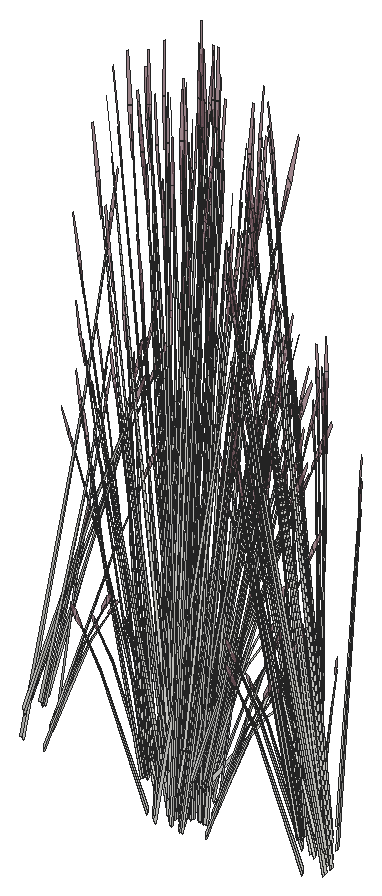
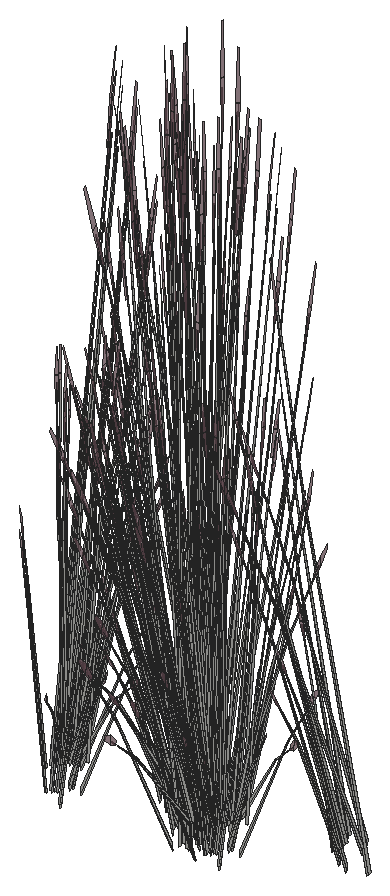
# SketchUp Ruby script. Lengths in inches.
U = 1.inch
M = Sketchup.active_model
def pt(a) = Geom::Point3d.new(a.map { |v| v * U })
def face(e, loops, mat)
  f = e.add_face(loops[0].map { |a| pt(a) })
  loops[1..].each { |l| e.add_face(l.map { |a| pt(a) }).erase! }
  f.material = f.back_material = mat if mat
  f
end
# faces: each face lists its corners as indices into pts; further lists are holes
def faces(e, pts, list, mat = nil) = list.each { |f| face(e, (f[0].is_a?(Array) ? f : [f]).map { |l| l.map { |i| pts[i] } }, mat) }
# xy, xz, yz: faces in a plane at the given z, y or x. An outline is a flat list of corners, or four numbers for a rectangle; further outlines are holes
def ring(l) = l.size == 4 ? [[l[0], l[1]], [l[2], l[1]], [l[2], l[3]], [l[0], l[3]]] : l.each_slice(2).to_a
def flat(e, list, mat, &to3) = list.each { |f| face(e, (f[0].is_a?(Array) ? f : [f]).map { |l| ring(l).map { |u, v| to3.(u, v) } }, mat) }
def xy(e, z, list, mat = nil) = flat(e, list, mat) { |x, y| [x, y, z] }
def xz(e, y, list, mat = nil) = flat(e, list, mat) { |x, z| [x, y, z] }
def yz(e, x, list, mat = nil) = flat(e, list, mat) { |y, z| [x, y, z] }
def lines(e, pts, list) = list.each { |a, b| e.add_line(pt(pts[a]), pt(pts[b])) }
# prism: a flat outline (further loops are holes) pulled along v
def prism(e, loops, v, mat = nil)
  f = face(e, loops, mat); d = Geom::Vector3d.new(v.map { |x| x * U })
  f.pushpull(f.normal.samedirection?(d) ? d.length : -d.length)
end
def box(e, o, s, mat = nil) = prism(e, [[o, [o[0] + s[0], o[1], o[2]], [o[0] + s[0], o[1] + s[1], o[2]], [o[0], o[1] + s[1], o[2]]]], [0, 0, s[2]], mat)
def at(x, y, z, deg = 0) = Geom::Transformation.translation(pt([x, y, z])) * Geom::Transformation.rotation(ORIGIN, Z_AXIS, deg.degrees)
def axes(o, x, y, z) = Geom::Transformation.new([*x, 0, *y, 0, *z, 0, *pt(o).to_a, 1])
def part(name) = M.definitions.add(name)
# library, detail: a bought-in or finely detailed component or shape, given as its bounding box
def library(name, o, s) = part(name).tap { |d| box(d.entities, o, s) }
def detail(e, o, s) = box(e.add_group.entities, o, s)
def put(e, d, t, mat = nil) = e.add_instance(d, t).tap { |i| i.material = mat if mat }
def group(e, t, mat = nil) = e.add_group.tap { |g| g.transformation = t; g.material = mat if mat }.entities
root = M.entities
M.materials.add("LightPink_Translucent").color = [144, 107, 117]
M.materials["LightPink_Translucent"].alpha = 0.75
c1 = part("blade")
p = [[2.15,0.21,22],[0,0.17,0],[0.09,0.45,0],[2.18,0.31,22],[2.29,0.31,22],[0.38,0.45,0],
  [2.48,0.24,33],[2.49,0.24,33],[2.48,0.22,33]]
faces(c1.entities,p,[[0,1,2,3],[4,5,2,3],[6,3,4,7],[8,0,3,6]])
c2 = part("seeds")
p = [[0.3,-0.1,1.38],[-0.01,-0.03,1.59],[-0.01,-0.03,0.03],[0.14,-0.07,-0.07],[0.29,-0.03,3],[0.15,0.01,3.11]]
faces(c2.entities,p,[[0,1,2,3],[1,0,4,5]],"LightPink_Translucent")
c3 = part("blade with seeds")
put(c3.entities,c1,at(0,0,0))
put(c3.entities,c2,axes([2.4,0.25,30.99],[1.5799,-0.05474,1.17369],[-0.12525,1.92788,0.29478],[-0.07173,-0.02425,1.56792]))
put(root,c3,axes([249.3,462.4375,653.93],[-0.09617,-0.45271,-0.03492],[0.45453,-0.10408,-0.15832],[0.09492,0.0287,0.52218]))
put(root,c3,axes([247.53,460.36,652.06],[0.52267,0.08829,-0.62353],[-0.11029,0.54463,-0.16365],[0.15598,0.06599,1.37633]))
put(root,c3,axes([247.42,461.52,653.875],[-0.18664,-0.09279,1.71376],[0.38624,-0.38925,0.13857],[0.24072,0.1756,0.73262]))
put(root,c3,axes([248.45,462.39,654.53],[0.28589,0.33718,-0.35414],[-0.32644,0.31919,0.4572],[0.16586,0.04856,0.87481]))
put(root,c3,axes([249.84,461.31,652.77],[-0.31044,0.08891,1.1486],[0.14613,-0.36744,0.84392],[0.16469,0.02514,0.25299]))
put(root,c3,axes([248.95,461.22,654.53],[0.41757,0.15024,-0.35414],[-0.12179,0.4383,0.4572],[0.16812,-0.04019,0.87481]))
put(root,c3,axes([248.15,462.16,654.98],[0.50227,0.01297,-0.71045],[-0.03373,0.54602,0.08574],[0.21278,0.05762,1.00501]))
put(root,c3,axes([249.52,460.8,651.49],[-0.02626,-0.08176,1.76342],[0.18213,-0.47826,-0.26939],[0.18372,-0.00688,0.30037]))
put(root,c3,axes([247.82,460.67,653.875],[-0.20841,0.0122,1.71376],[0.13825,-0.52864,0.13857],[0.297,0.0327,0.73262]))
put(root,c3,axes([248.58,461.17,654.98],[0.44151,-0.23785,-0.71045],[0.24605,0.4896,0.08574],[0.21333,-0.05562,1.00501]))
put(root,c3,axes([249.26,461.9,652.59],[-0.12101,-0.13245,1.43002],[0.15744,-0.43816,-0.30754],[0.24483,0.05936,0.61141]))
put(root,c3,axes([259.18,461,651.875],[0.17434,-0.11391,1.71376],[0.14677,0.52637,0.13857],[-0.27369,0.11897,0.73262]))
put(root,c3,axes([258.63,461.89,650.59],[0.17462,0.04421,1.43002],[0.11254,0.45156,-0.30754],[-0.23719,0.08453,0.61141]))
put(root,c3,axes([260.18,460.45,651.34],[0.14282,-0.0779,1.77064],[0.04925,0.54394,0.13857],[-0.30935,0.07218,0.63284]))
put(root,c3,axes([258.64,460.8125,652.72],[-0.08205,0.06992,1.74944],[0.00698,0.51086,-0.27667],[-0.18807,0.06644,0.14031]))
put(root,c3,axes([258.9,460.52,652.53],[-0.41757,-0.15024,-0.35414],[0.12179,-0.4383,0.4572],[-0.16812,0.04019,0.87481]))
put(root,c3,axes([257.73,461.33,652.71],[0.06412,0.01444,1.77383],[0.19837,0.47583,-0.16761],[-0.13126,0.12489,0.31391]))
put(root,c3,axes([259.19,460.74,652.68],[-0.13612,0.48987,-0.51099],[-0.46669,-0.16791,-0.3958],[-0.1879,0.04492,0.97773]))
put(root,c3,axes([258.96,460.71,649.49],[0.01274,0.08487,1.76342],[-0.25688,0.44323,-0.26939],[-0.18246,-0.02234,0.30037]))
put(root,c3,axes([258.27,462.84,650.77],[0.2094,-0.24408,1.1486],[0.08263,0.38639,0.84392],[-0.15132,0.06919,0.25299]))
put(root,c3,axes([259,460.46,652.73],[0.14195,-0.49104,0.48003],[0.46669,0.16791,0.3958],[-0.18353,0.02951,0.9933]))
put(root,c3,axes([259.17,460.32,653.03],[0.25281,0.48765,-0.1216],[-0.44869,0.23964,-0.67495],[-0.18908,0.06434,1.02557]))
put(root,c3,axes([258.97,460.33,652.73],[-0.18454,-0.3672,0.0643],[0.33652,-0.17973,0.50621],[-0.14834,0.03546,0.77189]))
put(root,c3,axes([259.8125,461.35,651.875],[0.1255,-0.16547,1.71376],[0.31687,0.44665,0.13857],[-0.21734,0.2034,0.73262]))
put(root,c3,axes([259.06,461.78,652.53],[-0.43736,0.07697,-0.35414],[-0.11549,-0.43998,0.4572],[-0.12533,0.11818,0.87481]))
put(root,c3,axes([258.82,463.09,649.49],[0.0674,0.0538,1.76342],[0.11428,0.49852,-0.26939],[-0.14937,0.10631,0.30037]))
put(root,c3,axes([259.11,461.6875,652.73],[-0.12461,-0.49565,0.48003],[0.48882,-0.08602,0.3958],[-0.14406,0.11657,0.9933]))
put(root,c3,axes([259.02,461.59,652.73],[-0.34493,-0.22649,0.0643],[0.20082,-0.32253,0.50621],[-0.11059,0.10427,0.77189]))
put(root,c3,axes([259.72,461.76,651.875],[0.09355,-0.18511,1.71376],[0.39247,0.38307,0.13857],[-0.17705,0.23875,0.73262]))
put(root,c3,axes([259.34,460.47,653.05],[0.41757,0.15024,0.35414],[-0.12179,0.4383,-0.4572],[-0.16812,0.04019,0.87481]))
put(root,c3,axes([259.42,461.83,652.68],[0.12908,0.49174,-0.51099],[-0.48882,0.08602,-0.3958],[-0.14008,0.13208,0.97773]))
put(root,c3,axes([258.65,462.72,652.72],[-0.01249,0.10657,1.74944],[0.35444,0.37075,-0.27667],[-0.09279,0.17532,0.14031]))
put(root,c3,axes([260.64,461.48,650.06],[-0.52267,-0.08829,-0.62353],[0.11029,-0.54463,-0.16365],[-0.15598,-0.06599,1.37633]))
put(root,c3,axes([259.95,462.51,650.02],[-0.47024,-0.26927,-0.49651],[0.28107,-0.48284,0],[-0.1071,-0.06133,1.57504]))
put(root,c3,axes([259.1875,461.48,653.03],[0.46478,0.29695,-0.1216],[-0.26776,0.43004,-0.67495],[-0.13131,0.14949,1.02557]))
put(root,c3,axes([260.24,462.84,650.375],[-0.31414,0.53965,0],[-0.52557,-0.30095,-0.51607],[-0.1197,-0.06854,1.63711]))
put(root,c3,axes([258.42,462.77,653.65],[0.44338,0.14375,-0.06488],[-0.13639,0.44245,-0.29416],[-0.07252,0.06718,0.97024]))
put(root,c3,axes([259.41,461.52,653.05],[0.43736,-0.07697,0.35414],[0.11549,0.43998,-0.4572],[-0.12533,0.11818,0.87481]))
put(root,c3,axes([259.66,463.62,650.59],[0.15856,-0.08496,1.43002],[0.39147,0.25616,-0.30754],[-0.11652,0.22165,0.61141]))
put(root,c3,axes([261.23,461.5625,650.67],[-0.5073,0.35754,-0.29095],[-0.33735,-0.5052,-0.50002],[-0.12516,-0.05131,1.59708]))
put(root,c3,axes([259.83,462.69,652.73],[-0.35779,-0.36745,0.48003],[0.37996,-0.3169,0.3958],[-0.066,0.17239,0.9933]))
put(root,c3,axes([260.08,462.3125,650.03],[-0.11803,-0.46926,-0.30978],[0.46876,-0.13325,0.30978],[-0.0945,-0.05411,1.38974]))
put(root,c3,axes([259.7,462.66,652.73],[-0.4129,-0.02509,0.0643],[0.01132,-0.37891,0.50621],[-0.04321,0.14514,0.77189]))
put(root,c3,axes([259.83,462.8,652.53],[-0.33997,0.28354,-0.35414],[-0.32182,-0.32376,0.4572],[-0.04897,0.1645,0.87481]))
put(root,c3,axes([261.57,461.95,650.06],[-0.33843,0.40479,-0.62353],[-0.42041,-0.36705,-0.16365],[-0.13561,0.10098,1.37633]))
put(root,c3,axes([258.62,463.8125,652.71],[0.057,-0.03251,1.77383],[0.47114,0.21627,-0.16761],[-0.01107,0.18007,0.31391]))
put(root,c3,axes([261.8,461.73,650.46],[-0.49063,-0.43346,-0.25192],[0.41285,-0.48673,0.5513],[-0.13212,0.05071,1.68216]))
put(root,c3,axes([260.05,462.5,653.34],[-0.01307,0.49815,-0.7886],[-0.55054,-0.03346,0.09517],[-0.0581,0.21104,1.11556]))
put(root,c3,axes([260.04,463.9,650.77],[-0.013,-0.32022,1.1486],[0.32493,0.22839,0.84392],[-0.0639,0.15263,0.25299]))
put(root,c3,axes([261.55,461.63,650.21],[-0.54562,0.03324,-0.44739],[-0.04934,-0.55185,0.21531],[-0.09768,0.05593,1.43643]))
put(root,c3,axes([260.51,462.56,650.48],[0.47024,0.26927,0.49651],[-0.28107,0.48284,0],[-0.1071,-0.06133,1.57504]))
put(root,c3,axes([259.87,463.2,651.36],[0.01104,-0.27801,1.54345],[0.49652,0.14685,0.21329],[-0.04302,0.2963,0.72882]))
put(root,c3,axes([261.18,461.72,650.62],[-0.09693,0.48062,0.1448],[-0.47357,-0.08343,-0.41347],[-0.08619,-0.04935,1.26744]))
put(root,c3,axes([262.125,463.06,650.02],[-0.47024,0.26927,-0.49651],[-0.28107,-0.48284,0],[-0.1071,0.06133,1.57504]))
put(root,c3,axes([262.16,462.91,650.19],[-0.31023,-0.54153,-0.05142],[0.52557,-0.30095,0.51607],[-0.12951,0.05156,1.6363]))
put(root,c3,axes([260.17,462.67,653],[0.35968,0.36185,-0.5672],[-0.37996,0.3169,-0.43934],[-0.05473,0.18385,1.08528]))
put(root,c3,axes([262.01,462.84,650.03],[-0.46876,-0.13325,-0.30978],[0.11803,-0.46926,0.30978],[-0.0945,0.05411,1.38974]))
put(root,c3,axes([260,462.4,653.05],[0.33997,-0.28354,0.35414],[0.32182,0.32376,-0.4572],[-0.04897,0.1645,0.87481]))
put(root,c3,axes([262.28,460.84,650.84],[-0.01373,-0.50706,1.41272],[0.62119,0.13144,0.59816],[-0.14692,0.27746,1.3335]))
put(root,c3,axes([259.79,462.48,653.4],[0.55221,0.02668,-0.13498],[-0.01509,0.50521,-0.74919],[-0.03836,0.19458,1.13838]))
put(root,c3,axes([259.77,463.21,650.82],[0.45645,-0.09537,0.06507],[0.10494,0.38421,-0.86304],[-0.02894,0.19449,0.7736]))
put(root,c3,axes([261.93,461.48,650.67],[0.05855,0.61451,-0.29095],[-0.60981,0.03716,-0.50002],[-0.10738,0.08185,1.59708]))
put(root,c3,axes([260.57,462.15,651.875],[-0.0123,-0.2067,1.71376],[0.53301,0.13712,0.13857],[-0.03297,0.29456,0.73262]))
put(root,c3,axes([261.03,461.26,650.36],[0.63506,0.11347,0.45755],[-0.12924,0.64083,0.17955],[-0.09281,-0.06188,1.58856]))
put(root,c3,axes([260.68,462.28,650.47],[0.53992,-0.14294,0.17642],[0.13332,0.53195,0.35086],[-0.04815,-0.07751,1.60407]))
put(root,c3,axes([261.38,462.37,650.2],[-0.50654,-0.24178,0],[0.24378,-0.50239,0],[0,0,1.62707]))
put(root,c3,axes([262.55,462.97,650.375],[0.31414,0.53965,0],[-0.52557,0.30095,-0.51607],[-0.1197,0.06854,1.63711]))
put(root,c3,axes([260.95,463.21,653.0625],[-0.4951,-0.14079,0.53283],[0.1693,-0.46287,0.43934],[0.02975,0.18203,1.10256]))
put(root,c3,axes([260.82,463.24,652.73],[-0.37023,0.18303,0.0643],[-0.18122,-0.33376,0.50621],[0.03575,0.14712,0.77189]))
put(root,c3,axes([262.29,462.3125,650.47],[0.14515,-0.53522,0.17642],[0.53115,0.15146,0.35086],[-0.09175,0.00261,1.60407]))
put(root,c3,axes([262.05,461.6,650.62],[0.37121,0.32357,0.1448],[-0.30963,0.36505,-0.41347],[-0.08619,0.04935,1.26744]))
put(root,c3,axes([261.91,461.2,650.3],[-0.46736,-0.46353,-0.06131],[0.46764,-0.46381,0],[-0.01632,-0.01619,1.75571]))
put(root,c3,axes([262.04,461.37,650.72],[0.54562,-0.03324,0.44739],[0.04934,0.55185,-0.21531],[-0.09768,0.05593,1.43643]))
put(root,c3,axes([262.17,462.63,650.33],[0.62903,0.17504,0.30756],[-0.15737,0.62568,-0.36492],[-0.10411,0.07831,1.64885]))
put(root,c3,axes([262.44,462.6,650.48],[0.47024,-0.26927,0.49651],[0.28107,0.48284,0],[-0.1071,0.06133,1.57504]))
put(root,c3,axes([261.49,462.16,650.2],[-0.16394,-0.4643,0],[0.46814,-0.1626,0],[0,0,1.54371]))
put(root,c3,axes([260.9,463.14,649.49],[0.08132,-0.0293,1.76342],[0.48914,0.1613,-0.26939],[0.0143,0.18179,0.30037]))
put(root,c3,axes([261.01,463.3,652.53],[-0.15148,0.41415,-0.35414],[-0.44193,-0.12079,0.4572],[0.04052,0.16674,0.87481]))
put(root,c3,axes([262.16,461.24,650.21],[-0.24378,0.48527,-0.44739],[-0.50654,-0.23354,0.21531],[0,0.11186,1.43643]))
put(root,c3,axes([260.69,464.04,652.72],[0.06369,0.08672,1.74944],[0.51399,0.03407,-0.27667],[0.05169,0.19126,0.14031]))
put(root,c3,axes([263.12,460.95,650.47],[-0.39477,-0.39228,0.17642],[0.39783,-0.38049,0.35086],[-0.0436,0.08011,1.60407]))
put(root,c3,axes([261.76,460.72,650.21],[0,-0.62313,0],[0.62828,0,0],[0,0,1.79456]))
put(root,c3,axes([262.07,460.97,650.29],[0,0.62282,-0.05637],[-0.62828,0,0],[0,0.01957,1.79368]))
put(root,c3,axes([260.96,462.87,653.05],[0.15148,-0.41415,0.35414],[0.44193,0.12079,-0.4572],[0.04052,0.16674,0.87481]))
put(root,c3,axes([260.74,459.52,650.47],[-0.14515,0.53522,0.17642],[-0.53115,-0.15146,0.35086],[0.09175,-0.00261,1.60407]))
put(root,c3,axes([261.77,462.18,650.29],[0.21845,0.61869,-0.06012],[-0.62418,0.21679,0],[0.00763,0.02161,1.72173]))
put(root,c3,axes([261.05,462.93,652.98],[0.23981,0.43789,-0.71045],[-0.49365,0.24404,0.08574],[0.05608,0.21158,1.00501]))
put(root,c3,axes([263.58,461.36,650.2],[-0.62797,-0.00431,-0.04976],[0,-0.6019,0.49943],[-0.01973,0.13702,1.58352]))
put(root,c3,axes([262.34,459.55,650.47],[-0.53992,0.14294,0.17642],[-0.13332,-0.53195,0.35086],[0.04815,0.07751,1.60407]))
put(root,c3,axes([261.55,464.34,653.65],[0.34721,-0.30895,-0.06488],[0.31814,0.33837,-0.29416],[0.0224,0.09588,0.97024]))
put(root,c3,axes([261.46,460.33,650.36],[-0.4166,0.48873,0.45755],[-0.49494,-0.43142,0.17955],[0.10044,-0.04877,1.58856]))
put(root,c3,axes([262.17,461.1,650.21],[0.35073,0.34786,0],[-0.35073,0.34786,0],[0,0,1.69266]))
put(root,c3,axes([262.17,460.69,650.72],[0.24378,-0.48527,0.44739],[0.50654,0.23354,-0.21531],[0,0.11186,1.43643]))
put(root,c3,axes([261.95,462.38,650.2],[0.50654,0.24178,0],[-0.24378,0.50239,0],[0,0,1.74954]))
put(root,c3,axes([261.23,463.02,652.68],[0.49392,0.135,-0.51099],[-0.1693,0.46287,-0.3958],[0.04529,0.18636,0.97773]))
put(root,c3,axes([260.81,463.04,653.03],[0.49168,-0.25073,-0.1216],[0.24162,0.44501,-0.67495],[0.06487,0.18753,1.02557]))
put(root,c3,axes([262,460.58,650.38],[-0.63506,-0.11347,0.49198],[0.12924,-0.64083,0.19306],[0.09281,0.06188,1.70813]))
put(root,c3,axes([263.45,461.45,650.03],[-0.35073,0.33601,-0.30978],[-0.35073,-0.33601,0.30978],[0,0.10823,1.38974]))
put(root,c3,axes([262.44,461.39,650.09],[0.18424,0.49308,-0.69212],[-0.53071,0.17758,-0.18165],[0.02036,0.16697,1.52773]))
put(root,c3,axes([262.18,460.86,650.21],[0.56215,0,0],[0,0.55754,0],[0,0,1.78407]))
put(root,c3,axes([261.64,460.25,650.72],[-0.30184,-0.45202,0.44739],[0.45719,-0.31831,-0.21531],[0.09768,0.05593,1.43643]))
put(root,c3,axes([262.38,460.8,650.62],[0.46814,-0.15705,0.1448],[0.16394,0.44848,-0.41347],[0,0.0987,1.26744]))
put(root,c3,axes([262.22,460.84,650.67],[0.56585,0.25696,-0.29095],[-0.27246,0.54236,-0.50002],[0.01778,0.13316,1.59708]))
put(root,c3,axes([263.45,460.96,650.48],[0,-0.53854,0.49651],[0.56215,0,0],[0,0.12266,1.57504]))
put(root,c3,axes([263.6875,461.46,650.02],[0,0.53854,-0.49651],[-0.56215,0,0],[0,0.12266,1.57504]))
put(root,c3,axes([262.19,463.09,652.73],[-0.49974,0.12359,0.48003],[-0.08673,-0.48481,0.3958],[0.11753,0.14288,0.9933]))
put(root,c3,axes([262.09,463.19,652.73],[-0.22836,0.34211,0.0643],[-0.3252,-0.19918,0.50621],[0.10513,0.10968,0.77189]))
put(root,c3,axes([261.51,462.0625,651.875],[-0.11485,-0.17291,1.71376],[0.53072,-0.14557,0.13857],[0.11995,0.27145,0.73262]))
put(root,c3,axes([261.84,460.12,650.62],[0.09693,-0.48062,0.1448],[0.47357,0.08343,-0.41347],[0.08619,0.04935,1.26744]))
put(root,c3,axes([262.52,459.28,650.48],[-0.47024,-0.26927,0.49651],[0.28107,-0.48284,0],[0.1071,0.06133,1.57504]))
put(root,c3,axes([262.11,462.09,650.18],[0.5275,-0.18273,-0.19198],[0.18536,0.52636,0.00008],[0.05823,-0.0202,1.73897]))
put(root,c3,axes([262.02,462.8,653.05],[-0.0776,-0.43378,0.35414],[0.44361,-0.11454,-0.4572],[0.11915,0.12431,0.87481]))
put(root,c3,axes([262.12,460.53,650.21],[0.30184,0.45202,-0.44739],[-0.45719,0.31831,0.21531],[0.09768,0.05593,1.43643]))
put(root,c3,axes([262.32,460.3,652.47],[-0.43417,-0.27982,1.38283],[0.45844,-0.43566,0.59665],[0.14008,0.26255,1.33663]))
put(root,c3,axes([261.59,463.4,652.71],[0.00149,-0.0652,1.77383],[0.43058,-0.28766,-0.16761],[0.14956,0.10267,0.31391]))
put(root,c3,axes([262.97,462.58,650.77],[-0.2829,-0.15485,1.1486],[0.36529,-0.15734,0.84392],[0.09853,0.13328,0.25299]))
put(root,c3,axes([261.97,462.41,650.59],[0.00887,-0.17852,1.43002],[0.42372,-0.19941,-0.30754],[0.1308,0.21367,0.61141]))
put(root,c3,axes([262.94,459.53,650.03],[0.11803,0.46926,-0.30978],[-0.46876,0.13325,0.30978],[0.0945,0.05411,1.38974]))
put(root,c3,axes([263.83,461.05,650.375],[0.62828,0,0],[0,0.6019,-0.51607],[0,0.13709,1.63711]))
put(root,c3,axes([261.8,460.27,650.67],[0.5073,-0.35754,-0.29095],[0.33735,0.5052,-0.50002],[0.12516,0.05131,1.59708]))
put(root,c3,axes([263.02,463.28,650.67],[-0.3222,-0.01689,1.0506],[0.21278,-0.35872,0.58006],[0.12729,0.12745,0.8241]))
put(root,c3,axes([261.98,463.02,653.03],[0.2994,-0.46097,-0.1216],[0.43359,0.26557,-0.67495],[0.15072,0.13024,1.02557]))
put(root,c3,axes([260.52,459.96,649.59],[-0.49456,0.21561,1.28929],[-0.15741,-0.61865,0.50096],[0.30369,0.01029,1.46642]))
put(root,c3,axes([262.33,462.79,652.68],[0.4958,-0.12802,-0.51099],[0.08673,0.48481,-0.3958],[0.13317,0.13893,0.97773]))
put(root,c3,axes([262.9,462.21,653.05],[-0.28589,-0.33718,0.35414],[0.32644,-0.31919,-0.4572],[0.16586,0.04856,0.87481]))
put(root,c3,axes([263.08,459.32,650.02],[0.47024,0.26927,-0.49651],[-0.28107,0.48284,0],[0.1071,0.06133,1.57504]))
put(root,c3,axes([263.16,462.52,652.73],[-0.0253,0.40952,0.0643],[-0.38204,-0.01123,0.50621],[0.14634,0.04285,0.77189]))
put(root,c3,axes([263.05,463.16,649.49],[0.03661,-0.07775,1.76342],[0.46087,-0.22898,-0.26939],[0.13972,0.11851,0.30037]))
put(root,c3,axes([263.2,462.39,652.73],[-0.37048,0.35486,0.48003],[-0.31952,-0.37685,0.3958],[0.17382,0.06546,0.9933]))
put(root,c3,axes([264.16,462.4375,651.93],[-0.09617,-0.45271,-0.03492],[0.45453,-0.10408,-0.15832],[0.09492,0.0287,0.52218]))
put(root,c3,axes([263.375,461.27,653.05],[-0.41757,-0.15024,0.35414],[0.12179,-0.4383,-0.4572],[0.16812,-0.04019,0.87481]))
put(root,c3,axes([262.39,460.36,650.06],[0.52267,0.08829,-0.62353],[-0.11029,0.54463,-0.16365],[0.15598,0.06599,1.37633]))
put(root,c3,axes([262.28,461.52,651.875],[-0.18664,-0.09279,1.71376],[0.38624,-0.38925,0.13857],[0.24072,0.1756,0.73262]))
put(root,c3,axes([263.75,461.4,652.73],[0.18454,0.3672,0.0643],[-0.33652,0.17973,0.50621],[0.14834,-0.03546,0.77189]))
put(root,c3,axes([263.31,462.39,652.53],[0.28589,0.33718,-0.35414],[-0.32644,0.31919,0.4572],[0.16586,0.04856,0.87481]))
put(root,c3,axes([262.98,462.43,653.03],[0.0269,-0.54769,-0.1216],[0.50939,0.01497,-0.67495],[0.19618,0.03804,1.02557]))
put(root,c3,axes([263.72,461.27,652.73],[-0.14195,0.49104,0.48003],[-0.46669,-0.16791,0.3958],[0.18353,-0.02951,0.9933]))
put(root,c3,axes([263.42,462.1,652.72],[0.10779,-0.00911,1.74944],[0.29564,-0.41839,-0.27667],[0.19172,0.05523,0.14031]))
put(root,c3,axes([264.7,461.31,650.77],[-0.31044,0.08891,1.1486],[0.14613,-0.36744,0.84392],[0.16469,0.02514,0.25299]))
put(root,c3,axes([263.8125,461.22,652.53],[0.41757,0.15024,-0.35414],[-0.12179,0.4383,0.4572],[0.16812,-0.04019,0.87481]))
put(root,c3,axes([263.01,462.16,652.98],[0.50227,0.01297,-0.71045],[-0.03373,0.54602,0.08574],[0.21278,0.05762,1.00501]))
put(root,c3,axes([264.38,460.8,649.49],[-0.02626,-0.08176,1.76342],[0.18213,-0.47826,-0.26939],[0.18372,-0.00688,0.30037]))
put(root,c3,axes([264.55,462.86,652.71],[-0.04543,-0.04715,1.77383],[0.09938,-0.50538,-0.16761],[0.17896,-0.03229,0.31391]))
put(root,c3,axes([262.68,460.67,651.875],[-0.20841,0.0122,1.71376],[0.13825,-0.52864,0.13857],[0.297,0.0327,0.73262]))
put(root,c3,axes([263.4375,461.17,652.98],[0.44151,-0.23785,-0.71045],[0.24605,0.4896,0.08574],[0.21333,-0.05562,1.00501]))
put(root,c3,axes([264.12,461.9,650.59],[-0.12101,-0.13245,1.43002],[0.15744,-0.43816,-0.30754],[0.24483,0.05936,0.61141]))
put(root,c3,axes([273.43,461,651.875],[0.17434,-0.11391,1.71376],[0.14677,0.52637,0.13857],[-0.27369,0.11897,0.73262]))
put(root,c3,axes([273.43,461,653.875],[0.17434,-0.11391,1.71376],[0.14677,0.52637,0.13857],[-0.27369,0.11897,0.73262]))
put(root,c3,axes([272.89,461.89,650.59],[0.17462,0.04421,1.43002],[0.11254,0.45156,-0.30754],[-0.23719,0.08453,0.61141]))
put(root,c3,axes([272.89,461.89,652.59],[0.17462,0.04421,1.43002],[0.11254,0.45156,-0.30754],[-0.23719,0.08453,0.61141]))
put(root,c3,axes([274.43,460.45,651.34],[0.14282,-0.0779,1.77064],[0.04925,0.54394,0.13857],[-0.30935,0.07218,0.63284]))
put(root,c3,axes([274.43,460.45,653.34],[0.14282,-0.0779,1.77064],[0.04925,0.54394,0.13857],[-0.30935,0.07218,0.63284]))
put(root,c3,axes([272.89,460.8125,652.72],[-0.08205,0.06992,1.74944],[0.00698,0.51086,-0.27667],[-0.18807,0.06644,0.14031]))
put(root,c3,axes([273.16,460.52,652.53],[-0.41757,-0.15024,-0.35414],[0.12179,-0.4383,0.4572],[-0.16812,0.04019,0.87481]))
put(root,c3,axes([273.16,460.52,654.53],[-0.41757,-0.15024,-0.35414],[0.12179,-0.4383,0.4572],[-0.16812,0.04019,0.87481]))
put(root,c3,axes([271.98,461.33,652.71],[0.06412,0.01444,1.77383],[0.19837,0.47583,-0.16761],[-0.13126,0.12489,0.31391]))
put(root,c3,axes([273.44,460.74,652.68],[-0.13612,0.48987,-0.51099],[-0.46669,-0.16791,-0.3958],[-0.1879,0.04492,0.97773]))
put(root,c3,axes([273.44,460.74,654.68],[-0.13612,0.48987,-0.51099],[-0.46669,-0.16791,-0.3958],[-0.1879,0.04492,0.97773]))
put(root,c3,axes([273.21,460.71,649.49],[0.01274,0.08487,1.76342],[-0.25688,0.44323,-0.26939],[-0.18246,-0.02234,0.30037]))
put(root,c3,axes([273.21,460.71,651.49],[0.01274,0.08487,1.76342],[-0.25688,0.44323,-0.26939],[-0.18246,-0.02234,0.30037]))
put(root,c3,axes([272.52,462.84,650.77],[0.2094,-0.24408,1.1486],[0.08263,0.38639,0.84392],[-0.15132,0.06919,0.25299]))
put(root,c3,axes([272.52,462.84,652.77],[0.2094,-0.24408,1.1486],[0.08263,0.38639,0.84392],[-0.15132,0.06919,0.25299]))
put(root,c3,axes([273.26,460.46,652.73],[0.14195,-0.49104,0.48003],[0.46669,0.16791,0.3958],[-0.18353,0.02951,0.9933]))
put(root,c3,axes([273.42,460.32,653.03],[0.25281,0.48765,-0.1216],[-0.44869,0.23964,-0.67495],[-0.18908,0.06434,1.02557]))
put(root,c3,axes([273.22,460.33,652.73],[-0.18454,-0.3672,0.0643],[0.33652,-0.17973,0.50621],[-0.14834,0.03546,0.77189]))
put(root,c3,axes([274.07,461.35,651.875],[0.1255,-0.16547,1.71376],[0.31687,0.44665,0.13857],[-0.21734,0.2034,0.73262]))
put(root,c3,axes([274.07,461.35,653.875],[0.1255,-0.16547,1.71376],[0.31687,0.44665,0.13857],[-0.21734,0.2034,0.73262]))
put(root,c3,axes([273.3125,461.78,652.53],[-0.43736,0.07697,-0.35414],[-0.11549,-0.43998,0.4572],[-0.12533,0.11818,0.87481]))
put(root,c3,axes([273.3125,461.78,654.53],[-0.43736,0.07697,-0.35414],[-0.11549,-0.43998,0.4572],[-0.12533,0.11818,0.87481]))
put(root,c3,axes([273.07,463.09,649.49],[0.0674,0.0538,1.76342],[0.11428,0.49852,-0.26939],[-0.14937,0.10631,0.30037]))
put(root,c3,axes([273.07,463.09,651.49],[0.0674,0.0538,1.76342],[0.11428,0.49852,-0.26939],[-0.14937,0.10631,0.30037]))
put(root,c3,axes([273.37,461.6875,652.73],[-0.12461,-0.49565,0.48003],[0.48882,-0.08602,0.3958],[-0.14406,0.11657,0.9933]))
put(root,c3,axes([273.27,461.59,652.73],[-0.34493,-0.22649,0.0643],[0.20082,-0.32253,0.50621],[-0.11059,0.10427,0.77189]))
put(root,c3,axes([273.97,461.76,651.875],[0.09355,-0.18511,1.71376],[0.39247,0.38307,0.13857],[-0.17705,0.23875,0.73262]))
put(root,c3,axes([273.97,461.76,653.875],[0.09355,-0.18511,1.71376],[0.39247,0.38307,0.13857],[-0.17705,0.23875,0.73262]))
put(root,c3,axes([273.6,460.47,653.05],[0.41757,0.15024,0.35414],[-0.12179,0.4383,-0.4572],[-0.16812,0.04019,0.87481]))
put(root,c3,axes([273.67,461.83,652.68],[0.12908,0.49174,-0.51099],[-0.48882,0.08602,-0.3958],[-0.14008,0.13208,0.97773]))
put(root,c3,axes([273.67,461.83,654.68],[0.12908,0.49174,-0.51099],[-0.48882,0.08602,-0.3958],[-0.14008,0.13208,0.97773]))
put(root,c3,axes([272.91,462.72,652.72],[-0.01249,0.10657,1.74944],[0.35444,0.37075,-0.27667],[-0.09279,0.17532,0.14031]))
put(root,c3,axes([274.89,461.48,650.06],[-0.52267,-0.08829,-0.62353],[0.11029,-0.54463,-0.16365],[-0.15598,-0.06599,1.37633]))
put(root,c3,axes([274.89,461.48,652.06],[-0.52267,-0.08829,-0.62353],[0.11029,-0.54463,-0.16365],[-0.15598,-0.06599,1.37633]))
put(root,c3,axes([274.2,462.51,650.02],[-0.47024,-0.26927,-0.49651],[0.28107,-0.48284,0],[-0.1071,-0.06133,1.57504]))
put(root,c3,axes([274.2,462.51,652.02],[-0.47024,-0.26927,-0.49651],[0.28107,-0.48284,0],[-0.1071,-0.06133,1.57504]))
put(root,c3,axes([273.44,461.48,653.03],[0.46478,0.29695,-0.1216],[-0.26776,0.43004,-0.67495],[-0.13131,0.14949,1.02557]))
put(root,c3,axes([274.49,462.84,650.375],[-0.31414,0.53965,0],[-0.52557,-0.30095,-0.51607],[-0.1197,-0.06854,1.63711]))
put(root,c3,axes([274.49,462.84,652.375],[-0.31414,0.53965,0],[-0.52557,-0.30095,-0.51607],[-0.1197,-0.06854,1.63711]))
put(root,c3,axes([272.68,462.77,653.65],[0.44338,0.14375,-0.06488],[-0.13639,0.44245,-0.29416],[-0.07252,0.06718,0.97024]))
put(root,c3,axes([273.67,461.52,653.05],[0.43736,-0.07697,0.35414],[0.11549,0.43998,-0.4572],[-0.12533,0.11818,0.87481]))
put(root,c3,axes([273.92,463.62,650.59],[0.15856,-0.08496,1.43002],[0.39147,0.25616,-0.30754],[-0.11652,0.22165,0.61141]))
put(root,c3,axes([273.92,463.62,652.59],[0.15856,-0.08496,1.43002],[0.39147,0.25616,-0.30754],[-0.11652,0.22165,0.61141]))
put(root,c3,axes([275.48,461.5625,650.67],[-0.5073,0.35754,-0.29095],[-0.33735,-0.5052,-0.50002],[-0.12516,-0.05131,1.59708]))
put(root,c3,axes([275.48,461.5625,652.67],[-0.5073,0.35754,-0.29095],[-0.33735,-0.5052,-0.50002],[-0.12516,-0.05131,1.59708]))
